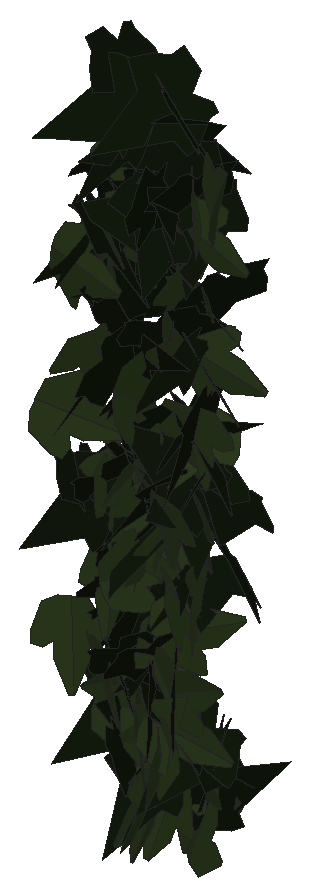
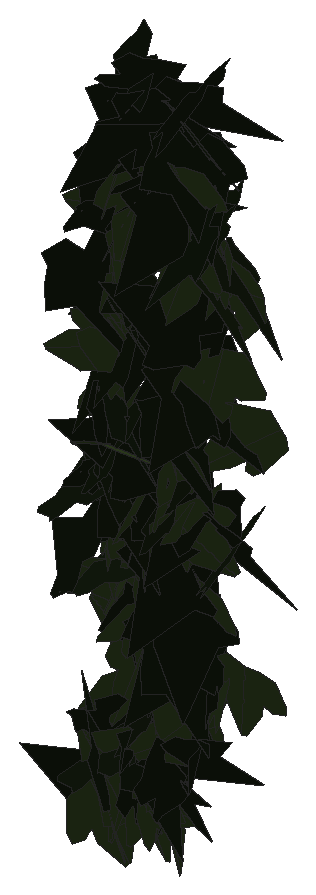
# SketchUp Ruby script. Lengths in inches.
U = 1.inch
M = Sketchup.active_model
def pt(a) = Geom::Point3d.new(a.map { |v| v * U })
def face(e, loops, mat)
  f = e.add_face(loops[0].map { |a| pt(a) })
  loops[1..].each { |l| e.add_face(l.map { |a| pt(a) }).erase! }
  f.material = f.back_material = mat if mat
  f
end
# faces: each face lists its corners as indices into pts; further lists are holes
def faces(e, pts, list, mat = nil) = list.each { |f| face(e, (f[0].is_a?(Array) ? f : [f]).map { |l| l.map { |i| pts[i] } }, mat) }
# xy, xz, yz: faces in a plane at the given z, y or x. An outline is a flat list of corners, or four numbers for a rectangle; further outlines are holes
def ring(l) = l.size == 4 ? [[l[0], l[1]], [l[2], l[1]], [l[2], l[3]], [l[0], l[3]]] : l.each_slice(2).to_a
def flat(e, list, mat, &to3) = list.each { |f| face(e, (f[0].is_a?(Array) ? f : [f]).map { |l| ring(l).map { |u, v| to3.(u, v) } }, mat) }
def xy(e, z, list, mat = nil) = flat(e, list, mat) { |x, y| [x, y, z] }
def xz(e, y, list, mat = nil) = flat(e, list, mat) { |x, z| [x, y, z] }
def yz(e, x, list, mat = nil) = flat(e, list, mat) { |y, z| [x, y, z] }
def lines(e, pts, list) = list.each { |a, b| e.add_line(pt(pts[a]), pt(pts[b])) }
# prism: a flat outline (further loops are holes) pulled along v
def prism(e, loops, v, mat = nil)
  f = face(e, loops, mat); d = Geom::Vector3d.new(v.map { |x| x * U })
  f.pushpull(f.normal.samedirection?(d) ? d.length : -d.length)
end
def box(e, o, s, mat = nil) = prism(e, [[o, [o[0] + s[0], o[1], o[2]], [o[0] + s[0], o[1] + s[1], o[2]], [o[0], o[1] + s[1], o[2]]]], [0, 0, s[2]], mat)
def at(x, y, z, deg = 0) = Geom::Transformation.translation(pt([x, y, z])) * Geom::Transformation.rotation(ORIGIN, Z_AXIS, deg.degrees)
def axes(o, x, y, z) = Geom::Transformation.new([*x, 0, *y, 0, *z, 0, *pt(o).to_a, 1])
def part(name) = M.definitions.add(name)
# library, detail: a bought-in or finely detailed component or shape, given as its bounding box
def library(name, o, s) = part(name).tap { |d| box(d.entities, o, s) }
def detail(e, o, s) = box(e.add_group.entities, o, s)
def put(e, d, t, mat = nil) = e.add_instance(d, t).tap { |i| i.material = mat if mat }
def group(e, t, mat = nil) = e.add_group.tap { |g| g.transformation = t; g.material = mat if mat }.entities
root = M.entities
M.materials.add("efeu1").color = [18, 25, 13]
M.materials.add("efeu2").color = [43, 57, 29]
c1 = part("ivyleaf_10")
p = [[0,0.5,-0.03],[-0.0625,2.02,-0.43],[-0.19,2.01,-0.46],[-0.54,1.05,-0.29],[-0.52,0.625,-0.18],[-0.83,0.76,-0.28],
  [-1.16,0.64,-0.33],[-1.15,0.33,-0.24],[-0.77,-0.39,0.02],[-0.3,-0.51,0.16],[0.04,-0.48,0.23],[-0.02,2.01,-0.4375],
  [-0.06,2.01,-0.43],[0.04,-0.49,0.23],[0.67,-0.49,0.14],[1.38,0.36,-0.2],[1.375,0.51,-0.24],[0.81,0.65,-0.19],
  [0.62,0.59,-0.15],[0.6,1.09,-0.28],[0.5,1.23,-0.31]]
faces(c1.entities,p,[[0,1,2,3,4,5,6,7,8,9,10],[11,12,0,13,14,15,16,17,18,19,20]],"efeu2")
c2 = part("ivyleaf_9")
p = [[1.54,2.16,1.25],[1.36,2.04,1.19],[-0.21,0.99,0.68],[-0.71,1.11,0.82],[-0.85,0.86,0.67],[-0.8,0.17,0.21],
  [-0.9,-0.01,0.1],[-0.67,-0.16,-0.02],[-0.08,-0.08,-0.05],[-0.03,-0.6,-0.4],[0.65,-0.88,-0.66],[0.83,-0.6,-0.49],
  [1.29,-0.42,-0.43],[1.8125,-0.07,-0.26],[1.21,0.44,0.15]]
faces(c2.entities,p,[[0,1,2,3,4,5,6,7,8,9,10,11,12,13,14]],"efeu1")
put(root,c1,axes([45.38,221.22,230.77],[-0.09708,-0.0266,-0.48976],[0.45063,-0.20197,-0.07836],[-0.19366,-0.45662,0.06319]))
put(root,c1,axes([47.17,221.15,224.92],[-0.24485,-0.0234,0.43532],[0.43418,0.03178,0.24592],[-0.03917,0.49844,0.00476]))
put(root,c1,axes([47.08,221.04,224.17],[0.1675,-0.07563,-0.465],[-0.40619,0.22682,-0.1832],[0.23865,0.43913,0.01455]))
put(root,c2,axes([45.82,221.15,231.6],[0.38344,-0.30873,-0.08753],[-0.0662,0.05734,-0.49227],[0.31399,0.3891,0.0031]))
put(root,c1,axes([47.37,221.46,226.46],[0.11119,-0.24346,0.42234],[0.30582,-0.3025,-0.25489],[0.37962,0.31499,0.08164]))
put(root,c1,axes([47.04,220.98,224.08],[0.1612,-0.35615,-0.31173],[-0.0115,0.32627,-0.37871],[0.47316,0.12927,0.097]))
put(root,c2,axes([46.6,221.47,224.93],[0.01303,-0.0776,-0.49377],[0.45789,-0.19621,0.04292],[-0.20042,-0.4533,0.06595]))
put(root,c1,axes([47.25,221.01,226.46],[0.31629,-0.35341,-0.1583],[0.16314,0.30698,-0.35938],[0.3512,0.17569,0.3095]))
put(root,c2,axes([46.93,221.41,225.37],[-0.0999,-0.00864,-0.48984],[0.47622,-0.11909,-0.09502],[-0.11503,-0.48553,0.03202]))
put(root,c1,axes([47,221.11,227.66],[-0.47485,0.1445,0.0603],[-0.05811,0.01617,-0.49635],[-0.1454,-0.47839,0.00143]))
put(root,c2,axes([46.91,220.97,225.57],[0.16627,0.46696,-0.06562],[-0.02575,-0.06049,-0.49566],[-0.47084,0.16821,0.00393]))
put(root,c2,axes([46.5,220.92,225.45],[0.35847,0.34688,0.03432],[0.0242,0.02435,-0.49882],[-0.34773,0.35928,0.00067]))
put(root,c2,axes([46.39,221.41,233.3],[-0.42866,-0.06645,0.24867],[-0.24517,-0.04172,-0.43377],[0.0784,-0.49381,0.00318]))
put(root,c1,axes([46.64,221.21,223.08],[0.17762,-0.45613,-0.10198],[-0.03363,0.09634,-0.48948],[0.46618,0.18074,0.00355]))
put(root,c1,axes([45.85,221.22,225.0625],[-0.35163,0.31611,-0.16258],[0.11978,-0.10993,-0.47283],[-0.33468,-0.37147,0.00158]))
put(root,c1,axes([47.08,221.02,224.46],[0.18038,0.09571,0.4564],[0.33279,0.31638,-0.19787],[-0.32667,0.37515,0.05043]))
put(root,c2,axes([46.42,221.37,233.11],[-0.46403,0.10463,-0.15404],[0.14158,-0.07045,-0.47433],[-0.12096,-0.48383,0.03576]))
put(root,c1,axes([46.57,220.91,229.24],[-0.07316,0.27357,0.41208],[-0.17779,0.37417,-0.27997],[-0.46156,-0.18749,0.04252]))
put(root,c1,axes([45.35,220.96,228.61],[0.09982,0.19101,0.45117],[0.2374,0.38391,-0.21506],[-0.42857,0.25715,-0.01405]))
put(root,c2,axes([45.71,221.18,231.19],[-0.33427,0.37171,-0.00965],[0.00482,-0.00865,-0.4999],[-0.37181,-0.3343,0.0022]))
put(root,c1,axes([46.48,220.91,226.51],[-0.03208,-0.06777,0.49435],[0.10843,0.48258,0.0732],[-0.48705,0.1119,-0.01626]))
put(root,c2,axes([46.85,220.91,231.9],[0.01063,0.00114,0.49989],[0.19528,0.46026,-0.0052],[-0.46017,0.19535,0.00934]))
put(root,c1,axes([46.64,221.54,223.2],[0.04077,-0.39051,0.30958],[0.11399,-0.29507,-0.38722],[0.48512,0.10215,0.06497]))
put(root,c2,axes([46.22,221.14,224.02],[0.34141,-0.20724,-0.30082],[-0.26361,0.14527,-0.39926],[0.25289,0.43122,-0.01007]))
put(root,c2,axes([46.62,221.47,227.55],[-0.42729,-0.22844,-0.12343],[0.1198,0.03742,-0.48399],[0.23036,-0.44319,0.02276]))
put(root,c2,axes([46.04,221.39,229.72],[0.20152,-0.14296,0.43469],[0.34827,-0.26017,-0.24702],[0.29681,0.40234,-0.00528]))
put(root,c2,axes([46.27,220.88,229.6875],[-0.05874,0.16056,-0.46986],[-0.18054,0.43385,0.17083],[0.46255,0.18972,0.00701]))
put(root,c1,axes([45.9375,221.39,226.35],[0.45946,-0.14385,0.13492],[0.12728,-0.045,-0.48143],[0.15065,0.47674,-0.00473]))
put(root,c1,axes([47.14,221.17,225.85],[0.12999,0.0291,-0.48193],[0.47605,0.07551,0.13296],[0.08052,-0.49341,-0.00807]))
put(root,c1,axes([46.56,221.19,227.01],[-0.24047,-0.16011,-0.40809],[0.41021,0.08197,-0.27388],[0.1546,-0.46653,0.09193]))
put(root,c2,axes([47.01,221.43,231.62],[-0.27115,0.07458,0.41342],[-0.4197,-0.02679,-0.27044],[-0.01819,-0.49368,0.07713]))
put(root,c1,axes([46.57,221.27,227.82],[-0.27016,0.41735,-0.05327],[0.03422,-0.0413,-0.49711],[-0.41934,-0.27224,-0.00625]))
put(root,c2,axes([45.78,221.41,227.3],[-0.4876,0.08547,0.07031],[-0.06685,0.02568,-0.49485],[-0.0882,-0.49197,-0.01362]))
put(root,c1,axes([45.26,221.37,225.32],[0.48093,0.0349,0.13224],[0.13202,0.00784,-0.48219],[-0.03573,0.49872,-0.00168]))
put(root,c2,axes([47.04,221.45,226.62],[-0.45652,0.11548,-0.16807],[0.1601,-0.05228,-0.47078],[-0.12631,-0.48366,0.01075]))
put(root,c2,axes([45.9375,221.43,229.36],[-0.28714,0.31168,-0.26534],[0.12632,-0.24082,-0.41958],[-0.38935,-0.30799,0.05956]))
put(root,c2,axes([46.69,221.65,231.87],[-0.1221,-0.47615,0.09148],[0.0173,-0.09856,-0.48989],[0.48455,-0.11647,0.04054]))
put(root,c2,axes([46.65,221.53,223.55],[-0.47577,-0.09002,-0.12466],[0.12639,0.00191,-0.48376],[0.08757,-0.49183,0.02094]))
put(root,c2,axes([47.03,221.61,233.54],[-0.43424,-0.17303,0.17746],[-0.16356,-0.06894,-0.46744],[0.18623,-0.46401,0.00328]))
put(root,c1,axes([45.77,221.33,231.2],[-0.4171,0.26595,-0.07279],[0.04738,-0.0609,-0.49401],[-0.27163,-0.419,0.02561]))
put(root,c1,axes([46.64,221.59,223.25],[0.08083,0.3336,-0.36357],[-0.1846,-0.32121,-0.33578],[-0.45759,0.18851,0.07124]))
put(root,c1,axes([47.07,221.53,230.9],[0.11064,-0.46952,0.13158],[0.04141,-0.12539,-0.48225],[0.48584,0.11761,0.01114]))
put(root,c2,axes([47.03,221.26,233.6],[0.4365,-0.13199,-0.20505],[-0.19223,0.07248,-0.45585],[0.15006,0.47679,0.01253]))
put(root,c2,axes([47,221.67,232.95],[-0.0662,-0.12625,-0.47925],[-0.19352,-0.43854,0.14226],[-0.45625,0.20432,0.0092]))
put(root,c1,axes([46.89,221.36,225.71],[0.14721,0.47777,-0.00828],[-0.00213,-0.00801,-0.49993],[-0.47783,0.14723,-0.00033]))
put(root,c1,axes([46.42,221.48,224.33],[-0.13016,0.43893,-0.201],[0.04495,-0.19626,-0.45767],[-0.48066,-0.13721,0.01163]))
put(root,c1,axes([45.77,221.32,229.59],[-0.27497,-0.38804,-0.15431],[0.08924,0.12589,-0.47559],[0.40795,-0.28909,0.00002]))
put(root,c1,axes([46.56,221.32,227.55],[-0.36725,-0.20734,-0.26859],[0.25948,0.0834,-0.41918],[0.21863,-0.44728,0.04634]))
put(root,c2,axes([47,221.58,227.81],[-0.20165,0.2666,-0.37183],[0.01154,-0.40326,-0.29538],[-0.45739,-0.12771,0.15648]))
put(root,c2,axes([47.37,221.6875,224.23],[-0.42731,-0.2523,0.06124],[-0.0529,-0.03087,-0.49623],[0.25418,-0.43057,-0.00031]))
put(root,c1,axes([46.82,221.48,223.2],[0.4791,-0.12174,-0.07513],[-0.07019,0.02879,-0.49421],[0.12466,0.4841,0.0105]))
put(root,c2,axes([47.27,221.63,227.8],[-0.20123,-0.45028,-0.08217],[-0.03377,-0.07491,0.4932],[-0.45647,0.20404,-0.00026]))
put(root,c2,axes([46.88,221.21,230.28],[0.26969,0.41385,-0.07744],[-0.04952,-0.06015,-0.49389],[-0.41811,0.27406,0.00855]))
put(root,c1,axes([46.23,221.8,227.76],[-0.00553,0.09918,-0.49003],[-0.06784,-0.48568,-0.09753],[-0.49535,0.0654,0.01883]))
put(root,c2,axes([47.22,221.52,230.02],[-0.45382,0.18224,-0.10409],[0.09556,-0.04136,-0.48904],[-0.18685,-0.46377,0.00271]))
put(root,c1,axes([46.61,221.52,226.73],[0.0962,-0.49058,0.00884],[0.00715,-0.00761,-0.49989],[0.49061,0.09631,0.00555]))
put(root,c2,axes([46.64,221.59,224.52],[0.28789,-0.3958,0.10231],[0.08231,-0.06645,-0.48868],[0.40043,0.29821,0.0269]))
put(root,c1,axes([46.96,221.55,227.17],[-0.06236,-0.49438,0.04127],[-0.00537,-0.04092,-0.49829],[0.49607,-0.0626,-0.00021]))
put(root,c2,axes([46.16,221.3125,232.6],[0.02806,0.48381,-0.12306],[-0.06516,-0.11865,-0.48133],[-0.49494,0.04305,0.05639]))
put(root,c1,axes([46.07,221.85,224.51],[-0.09314,-0.07573,-0.48538],[-0.19154,-0.44932,0.10686],[-0.45237,0.20585,0.05469]))
put(root,c2,axes([46.02,221.32,225.02],[0.28148,-0.00734,-0.41318],[-0.40936,0.0634,-0.28001],[0.0565,0.49591,0.02968]))
put(root,c2,axes([47.26,221.7,229.03],[-0.20149,0.20203,-0.41059],[0.29868,-0.28182,-0.28525],[-0.34668,-0.36022,-0.00711]))
put(root,c2,axes([47.22,221.55,232.34],[-0.09224,0.39903,-0.28682],[0.0354,-0.28568,-0.40882],[-0.49014,-0.09573,0.02445]))
put(root,c1,axes([46.69,221.68,226.27],[-0.2254,0.2727,-0.35332],[0.18998,-0.29955,-0.35239],[-0.40386,-0.2931,0.03142]))
put(root,c1,axes([47.1,221.68,232.28],[-0.15597,0.35558,-0.31502],[0.11316,-0.29421,-0.38812],[-0.46138,-0.19237,0.0113]))
put(root,c2,axes([46.54,221.51,225.25],[-0.37835,0.32535,-0.03167],[0.02354,-0.02119,-0.499],[-0.32604,-0.37908,0.00072]))
put(root,c1,axes([46.47,221.47,231.78],[-0.47693,0.14822,-0.02374],[0.02204,-0.00905,-0.49943],[-0.14849,-0.47744,0.0021]))
put(root,c1,axes([45.91,221.48,227.6],[-0.02015,0.49954,0.00722],[0.00724,0.00752,-0.49989],[-0.49954,-0.02004,-0.00754]))
put(root,c1,axes([47.15,221.63,231.6],[-0.15949,0.01729,-0.47357],[0.43993,-0.18032,-0.15474],[-0.17614,-0.46603,0.04231]))
put(root,c1,axes([47.13,221.55,228.79],[-0.49713,-0.01804,-0.0504],[0.05218,-0.05802,-0.49387],[0.01197,-0.49629,0.05957]))
put(root,c1,axes([46.1,221.62,232.34],[0.49306,-0.05348,-0.0635],[-0.06255,0.01217,-0.49592],[0.05459,0.49698,0.00531]))
put(root,c2,axes([45.96,221.26,227.7],[0.31494,0.37575,0.0981],[0.06385,0.07448,-0.49028],[-0.38306,0.32134,-0.00107]))
put(root,c1,axes([47.73,221.22,232.33],[0.04145,-0.00449,-0.49826],[-0.11834,0.48559,-0.01421],[0.48402,0.11911,0.03919]))
put(root,c1,axes([46.12,221.6875,228.41],[0.46019,-0.11537,0.15785],[0.14948,-0.0526,-0.47422],[0.12603,0.48366,-0.01392]))
put(root,c2,axes([47.09,221.77,227.97],[-0.1723,-0.44468,-0.15025],[0.0731,0.13268,-0.4765],[0.46365,-0.18617,0.01929]))
put(root,c2,axes([46.73,221.37,232.35],[0.31044,-0.0984,-0.3794],[-0.30431,0.24453,-0.31241],[0.24703,0.42488,0.09194]))
put(root,c1,axes([46.81,221.56,227.42],[-0.14718,0.47752,-0.01783],[0.00486,-0.01716,-0.49968],[-0.47782,-0.14726,0.00041]))
put(root,c2,axes([46.08,221.93,224.14],[-0.40373,-0.22839,0.18665],[-0.14863,-0.11576,-0.46315],[0.25477,-0.42946,0.02558]))
put(root,c2,axes([46.63,221.92,223.34],[0.03505,0.11327,0.48574],[-0.15326,-0.46093,0.11854],[0.47464,-0.1572,0.00241]))
put(root,c2,axes([45.86,221.41,230.82],[-0.21228,0.35338,0.28295],[-0.18585,0.21693,-0.41037],[-0.41279,-0.2794,0.03926]))
put(root,c2,axes([45.16,221.72,227.4],[0.2687,-0.41972,-0.04048],[-0.02078,0.03476,-0.49836],[0.42115,0.2695,0.00123]))
put(root,c1,axes([46.05,221.35,224.28],[0.11915,0.09016,0.47715],[0.26139,0.40215,-0.14126],[-0.40924,0.2831,0.0487]))
put(root,c1,axes([46.03,221.58,231.27],[-0.45713,-0.15837,-0.12631],[0.12259,0.03193,-0.48369],[0.16127,-0.47318,0.00963]))
put(root,c1,axes([46.91,221.62,225.08],[-0.4088,0.2711,-0.09688],[0.07618,-0.06039,-0.49046],[-0.27763,-0.41576,0.00807]))
put(root,c2,axes([47.13,221.74,227.9],[-0.3591,0.27421,-0.21414],[0.14398,-0.16303,-0.45021],[-0.31673,-0.38501,0.03813]))
put(root,c1,axes([47.15,221.68,222.47],[0.40105,-0.28471,-0.09002],[0.07312,-0.05251,0.49183],[-0.28951,-0.40766,-0.00048]))
put(root,c1,axes([46.96,221.73,229.65],[-0.18949,-0.46265,0.00681],[0.00896,0.00369,0.49991],[-0.46262,0.18957,0.00689]))
put(root,c2,axes([46,221.5625,227.78],[0.47575,-0.06011,0.14161],[0.14027,-0.01949,-0.47952],[0.06316,0.49599,-0.00168]))
put(root,c2,axes([47.09,221.58,228.73],[-0.30315,0.39761,0.00286],[-0.00059,0.00314,-0.49999],[-0.39762,-0.30315,-0.00144]))
put(root,c1,axes([46.76,221.61,223.87],[0.36762,0.24829,0.23066],[0.19288,0.12653,-0.44361],[-0.27866,0.41514,-0.00275]))
put(root,c1,axes([47.14,221.62,227.5625],[-0.37121,0.3344,-0.01954],[0.00634,-0.02214,-0.49947],[-0.33491,-0.37107,0.01219]))
put(root,c1,axes([45.95,221.81,227.51],[0.33939,0.19728,-0.30967],[-0.28265,-0.12879,-0.39182],[-0.23436,0.44102,0.0241]))
put(root,c2,axes([46.91,221.58,227.5],[-0.13334,0.4686,-0.11238],[0.01511,-0.11248,-0.48695],[-0.48165,-0.13326,0.01584]))
put(root,c2,axes([46.66,221.68,230.87],[0.4465,-0.2097,0.08163],[0.07256,-0.03753,-0.49328],[0.21301,0.45235,-0.00308]))
put(root,c2,axes([46.67,221.59,223.88],[-0.2009,0.45385,-0.0605],[0.03234,-0.05184,-0.49625],[-0.45672,-0.20331,-0.00853]))
put(root,c2,axes([46.99,222.05,226.45],[-0.12509,-0.45647,0.1612],[0.234,-0.20276,-0.3926],[0.42379,-0.02278,0.26435]))
put(root,c2,axes([46.76,221.4375,232.9375],[0.42282,0.22758,0.13939],[0.12218,0.0671,-0.48018],[-0.23727,0.44012,0.00114]))
put(root,c2,axes([46.04,221.88,227.78],[0.2864,-0.36771,0.18102],[0.1225,-0.13394,-0.46589],[0.39111,0.31121,0.01337]))
put(root,c2,axes([45.78,221.77,233.77],[0.19529,-0.4329,-0.15641],[-0.06413,0.14265,-0.47491],[0.45579,0.20555,0.00019]))
put(root,c2,axes([47.07,222.09,223.7],[-0.12714,-0.37807,0.3015],[0.23708,-0.32044,-0.30185],[0.42146,0.0662,0.26074]))
put(root,c2,axes([46.09,221.53,226.1],[0.18311,0.44699,-0.1291],[-0.10383,-0.09597,-0.47959],[-0.45353,0.20245,0.05768]))
put(root,c2,axes([46.21,221.7,229.0625],[-0.17361,0.4358,-0.17303],[0.051,-0.16587,-0.46892],[-0.46611,-0.18047,0.01314]))
put(root,c1,axes([47.13,221.73,230.45],[-0.43128,0.21053,-0.14026],[-0.12648,0.06065,0.47992],[0.21909,0.44944,0.00094]))
put(root,c2,axes([47.16,221.83,223.33],[-0.02427,0.3228,0.38107],[0.02307,-0.38039,0.32369],[0.49888,0.0333,0.00357]))
put(root,c1,axes([46.97,222.12,228.4],[-0.49828,-0.03266,0.02559],[0.02432,-0.47979,-0.13862],[0.03361,-0.13689,0.47972]))
put(root,c2,axes([45.95,221.56,230.16],[0.051,-0.07145,0.49223],[0.46681,0.17772,-0.02257],[-0.17173,0.46186,0.08483]))
put(root,c2,axes([46.18,221.45,226.72],[0.27269,0.40435,0.11019],[0.04234,0.10421,-0.48718],[-0.41695,0.27503,0.0226]))
put(root,c2,axes([47.1,221.61,223.07],[0.05133,-0.03067,0.49641],[0.49437,0.0578,-0.04754],[-0.05447,0.4957,0.03626]))
put(root,c2,axes([46.16,221.72,225.62],[-0.15701,0.44835,-0.15599],[0.0606,-0.14402,-0.47496],[-0.47082,-0.16805,-0.00911]))
put(root,c2,axes([46.98,222.04,231.9375],[-0.15105,-0.47606,-0.02336],[0.0088,0.02172,-0.49945],[0.47656,-0.1513,0.00181]))
put(root,c2,axes([46.09,222.14,223.71],[0.00345,0.01083,0.49987],[-0.25904,-0.42752,0.01105],[0.42765,-0.25905,0.00266]))
put(root,c1,axes([46.68,221.71,232.13],[-0.321,-0.35378,-0.14764],[0.09529,0.11289,-0.47768],[0.37132,-0.33481,-0.00505]))
put(root,c1,axes([47.22,221.9375,223.1875],[-0.21469,-0.41258,0.18354],[-0.08196,-0.16425,-0.46509],[0.44406,-0.22978,0.00289]))
put(root,c1,axes([47.0625,221.69,223.6],[-0.43956,0.21566,0.1014],[-0.09356,0.03951,-0.48958],[-0.21917,-0.44937,0.00562]))
put(root,c2,axes([46.12,221.53,231.97],[0.39689,0.29955,0.05242],[0.04285,0.03025,-0.49724],[-0.30107,0.3992,-0.00166]))
put(root,c1,axes([47.125,221.81,229.67],[-0.16899,-0.02573,-0.46987],[0.46742,-0.06691,-0.16445],[-0.05442,-0.49483,0.04667]))
put(root,c2,axes([46.86,222.04,228.39],[0.21661,-0.38782,0.2295],[0.11742,-0.19727,-0.44418],[0.43508,0.24633,0.00562]))
put(root,c1,axes([46.96,221.81,223.14],[-0.37908,-0.20716,0.25176],[0.22939,0.1049,0.43171],[-0.23169,0.44281,0.01551]))
put(root,c2,axes([47.5,221.82,230.86],[-0.05219,0.41437,-0.27491],[0.02488,-0.2739,-0.41756],[-0.49665,-0.05727,0.00797]))
put(root,c2,axes([47.37,222.09,226.63],[0.15655,-0.31141,0.35849],[0.17256,-0.31435,-0.34843],[0.44239,0.23282,0.00905]))
put(root,c2,axes([47,221.71,229.8125],[0.43673,-0.12433,-0.2093],[-0.20389,0.04811,-0.454],[0.13303,0.4819,-0.00867]))
put(root,c2,axes([47.34,222.19,227.56],[-0.13725,-0.39264,0.27747],[0.19826,-0.3091,-0.33933],[0.43801,0.01687,0.24054]))
put(root,c2,axes([45.93,221.44,229.29],[0.17504,0.40708,0.23162],[0.04604,0.23111,-0.44099],[-0.46609,0.1757,0.04342]))
put(root,c2,axes([46.03,221.5,225.6875],[0.32914,0.35642,0.12096],[0.04311,0.12393,-0.48248],[-0.37391,0.32803,0.05085]))
put(root,c2,axes([45.61,221.76,231.89],[0.43768,-0.20209,-0.13264],[-0.12101,0.05434,-0.48208],[0.20926,0.4541,-0.00134]))
put(root,c2,axes([46.43,221.71,228.25],[0.23366,-0.12024,0.42538],[0.44152,0.08692,-0.21796],[-0.02154,0.47748,0.14679]))
